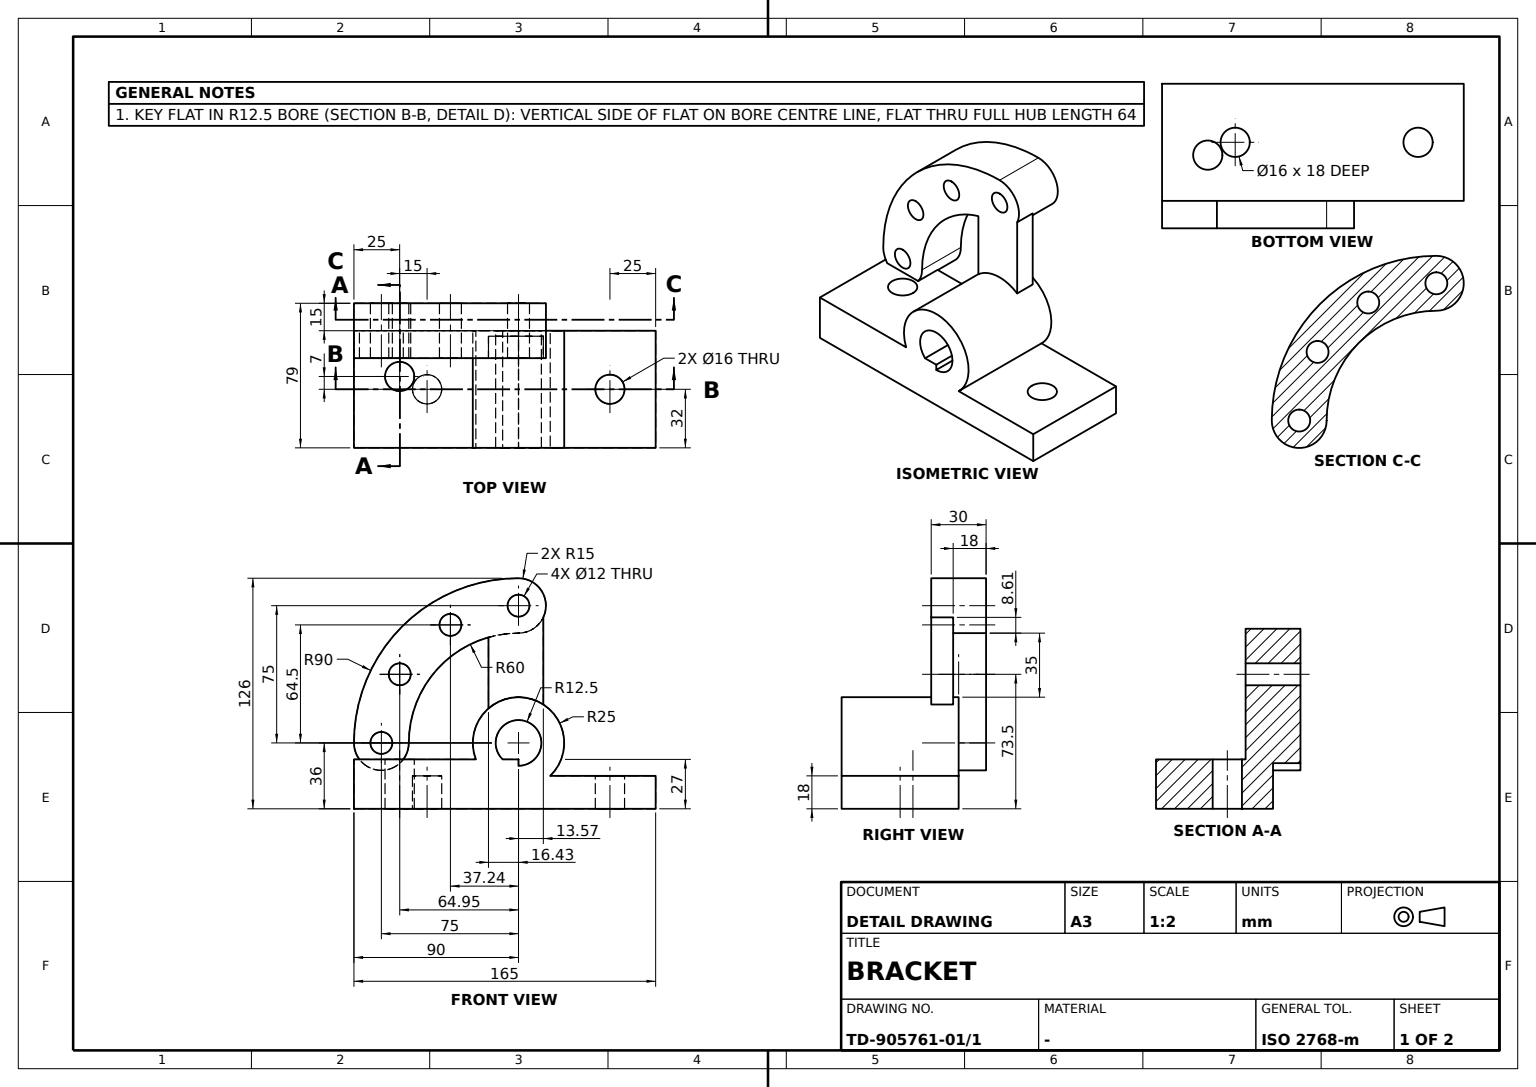
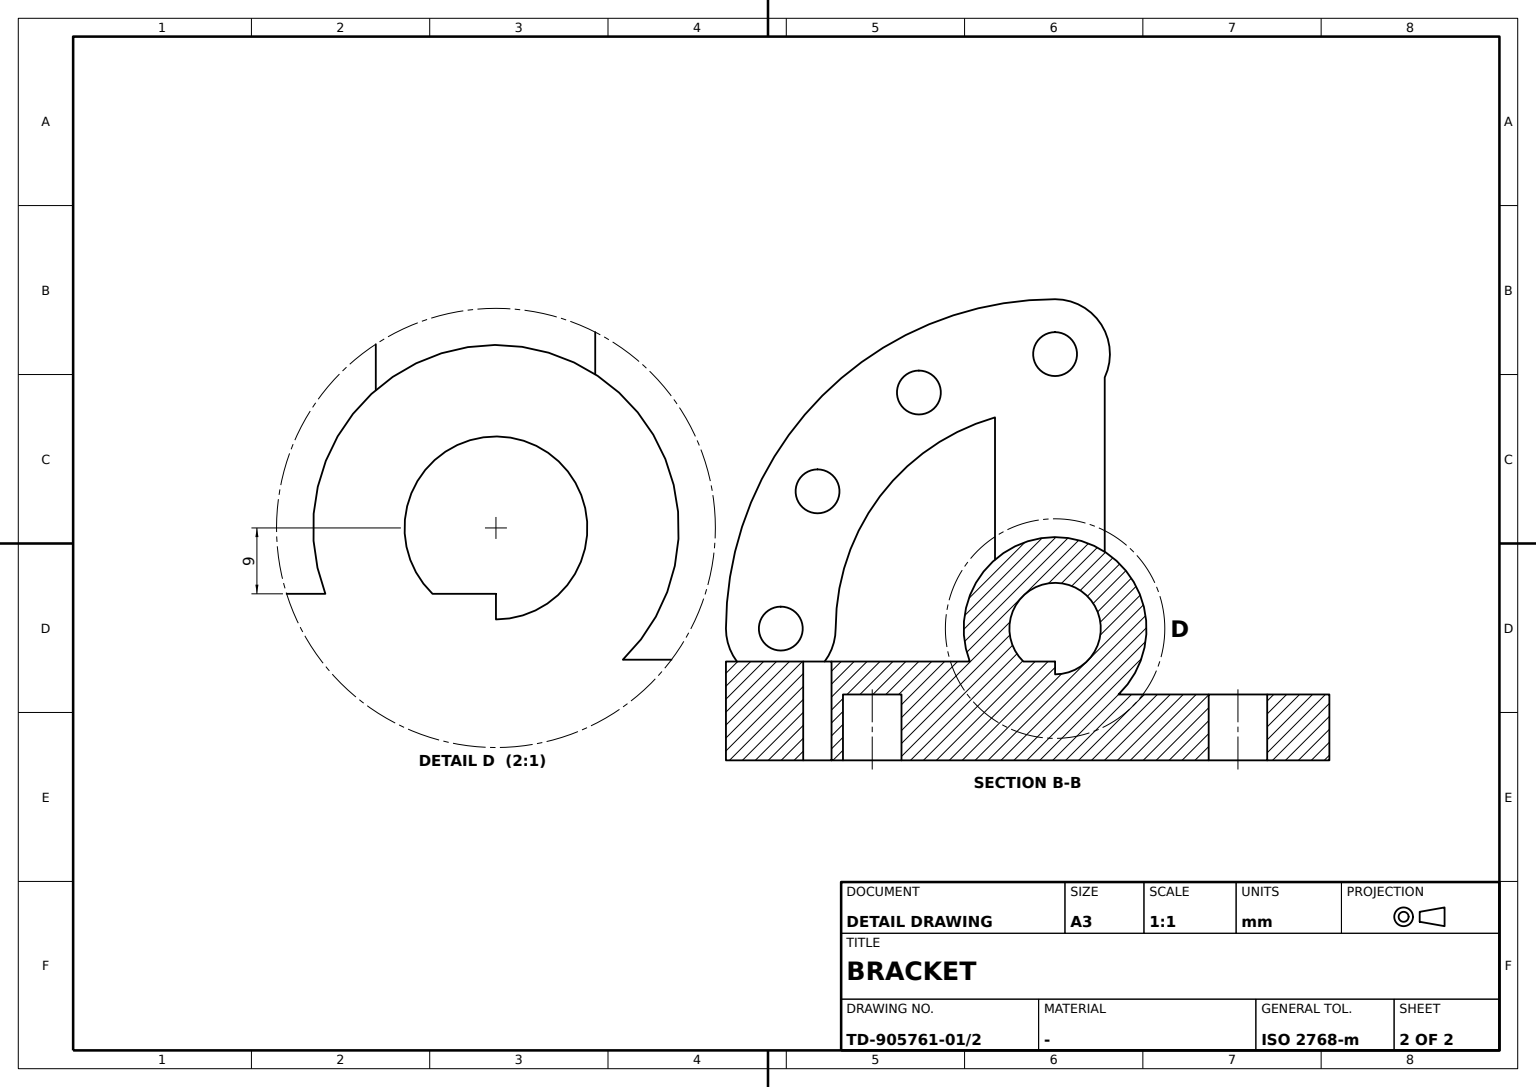
ISO-10303-21;
HEADER;
FILE_DESCRIPTION((''),'2;1');
FILE_NAME('','',(''),(''),'','','');
FILE_SCHEMA(('AUTOMOTIVE_DESIGN'));
ENDSEC;
DATA;
#1=APPLICATION_CONTEXT('');
#2=PRODUCT_CONTEXT('',#1,'mechanical');
#3=PRODUCT('','','',(#2));
#4=PRODUCT_DEFINITION_FORMATION('','',#3);
#5=PRODUCT_DEFINITION_CONTEXT('',#1,'design');
#6=PRODUCT_DEFINITION('','',#4,#5);
#7=PRODUCT_DEFINITION_SHAPE('','',#6);
#8=(LENGTH_UNIT()NAMED_UNIT(*)SI_UNIT(.MILLI.,.METRE.));
#9=(NAMED_UNIT(*)PLANE_ANGLE_UNIT()SI_UNIT($,.RADIAN.));
#10=(NAMED_UNIT(*)SI_UNIT($,.STERADIAN.)SOLID_ANGLE_UNIT());
#11=UNCERTAINTY_MEASURE_WITH_UNIT(LENGTH_MEASURE(0.005),#8,'distance_accuracy_value','');
#12=(GEOMETRIC_REPRESENTATION_CONTEXT(3)GLOBAL_UNCERTAINTY_ASSIGNED_CONTEXT((#11))GLOBAL_UNIT_ASSIGNED_CONTEXT((#8,#9,#10))REPRESENTATION_CONTEXT('',''));
#13=CARTESIAN_POINT('',(-16.427137,29.,57.707445));
#14=VERTEX_POINT('',#13);
#15=CARTESIAN_POINT('',(-16.427137,29.,18.845402));
#16=VERTEX_POINT('',#15);
#17=DIRECTION('',(0.,0.,-1.));
#18=VECTOR('',#17,1000.);
#19=LINE('',#13,#18);
#20=EDGE_CURVE('',#14,#16,#19,.T.);
#21=ORIENTED_EDGE('',*,*,#20,.F.);
#22=CARTESIAN_POINT('',(0.,29.,60.));
#23=VERTEX_POINT('',#22);
#24=CARTESIAN_POINT('',(0.,29.,0.));
#25=DIRECTION('',(0.,-1.,0.));
#26=AXIS2_PLACEMENT_3D('',#24,#25,#17);
#27=CIRCLE('',#26,60.);
#28=EDGE_CURVE('',#23,#14,#27,.T.);
#29=ORIENTED_EDGE('',*,*,#28,.F.);
#30=CARTESIAN_POINT('',(13.572863,29.,68.614283));
#31=VERTEX_POINT('',#30);
#32=CARTESIAN_POINT('',(0.,29.,75.));
#33=AXIS2_PLACEMENT_3D('',#32,#25,#17);
#34=CIRCLE('',#33,15.);
#35=EDGE_CURVE('',#23,#31,#34,.T.);
#36=ORIENTED_EDGE('',*,*,#35,.T.);
#37=CARTESIAN_POINT('',(13.572863,29.,20.994699));
#38=VERTEX_POINT('',#37);
#39=LINE('',#30,#18);
#40=EDGE_CURVE('',#31,#38,#39,.T.);
#41=ORIENTED_EDGE('',*,*,#40,.T.);
#42=CIRCLE('',#26,25.);
#43=EDGE_CURVE('',#38,#16,#42,.T.);
#44=ORIENTED_EDGE('',*,*,#43,.T.);
#45=EDGE_LOOP('',(#21,#29,#36,#41,#44));
#46=FACE_BOUND('',#45,.T.);
#47=DIRECTION('',(1.,0.,0.));
#48=AXIS2_PLACEMENT_3D('',#24,#25,#47);
#49=PLANE('',#48);
#50=ADVANCED_FACE('',(#46),#49,.F.);
#51=ORIENTED_EDGE('',*,*,#28,.T.);
#52=CARTESIAN_POINT('',(-16.427137,17.,57.707445));
#53=VERTEX_POINT('',#52);
#54=DIRECTION('',(0.,1.,0.));
#55=VECTOR('',#54,1000.);
#56=LINE('',#52,#55);
#57=EDGE_CURVE('',#53,#14,#56,.T.);
#58=ORIENTED_EDGE('',*,*,#57,.F.);
#59=CARTESIAN_POINT('',(-60.,17.,0.));
#60=VERTEX_POINT('',#59);
#61=CARTESIAN_POINT('',(0.,17.,0.));
#62=DIRECTION('',(0.,0.,1.));
#63=AXIS2_PLACEMENT_3D('',#61,#54,#62);
#64=CIRCLE('',#63,60.);
#65=EDGE_CURVE('',#60,#53,#64,.T.);
#66=ORIENTED_EDGE('',*,*,#65,.F.);
#67=CARTESIAN_POINT('',(-60.,47.,0.));
#68=VERTEX_POINT('',#67);
#69=CARTESIAN_POINT('',(-60.,32.,0.));
#70=LINE('',#69,#55);
#71=EDGE_CURVE('',#60,#68,#70,.T.);
#72=ORIENTED_EDGE('',*,*,#71,.T.);
#73=CARTESIAN_POINT('',(0.,47.,60.));
#74=VERTEX_POINT('',#73);
#75=CARTESIAN_POINT('',(0.,47.,0.));
#76=AXIS2_PLACEMENT_3D('',#75,#54,#62);
#77=CIRCLE('',#76,60.);
#78=EDGE_CURVE('',#68,#74,#77,.T.);
#79=ORIENTED_EDGE('',*,*,#78,.T.);
#80=CARTESIAN_POINT('',(0.,38.,60.));
#81=LINE('',#80,#55);
#82=EDGE_CURVE('',#23,#74,#81,.T.);
#83=ORIENTED_EDGE('',*,*,#82,.F.);
#84=EDGE_LOOP('',(#51,#58,#66,#72,#79,#83));
#85=FACE_BOUND('',#84,.T.);
#86=CARTESIAN_POINT('',(0.,32.,0.));
#87=DIRECTION('',(-1.,0.,0.));
#88=AXIS2_PLACEMENT_3D('',#86,#54,#87);
#89=CYLINDRICAL_SURFACE('',#88,60.);
#90=ADVANCED_FACE('',(#85),#89,.F.);
#91=CARTESIAN_POINT('',(-37.239092,17.,70.5));
#92=VERTEX_POINT('',#91);
#93=CARTESIAN_POINT('',(-37.239092,17.,64.5));
#94=AXIS2_PLACEMENT_3D('',#93,#54,#62);
#95=CIRCLE('',#94,6.);
#96=EDGE_CURVE('',#92,#92,#95,.T.);
#97=ORIENTED_EDGE('',*,*,#96,.F.);
#98=EDGE_LOOP('',(#97));
#99=FACE_BOUND('',#98,.T.);
#100=CARTESIAN_POINT('',(-37.239092,47.,70.5));
#101=VERTEX_POINT('',#100);
#102=CARTESIAN_POINT('',(-37.239092,47.,64.5));
#103=AXIS2_PLACEMENT_3D('',#102,#54,#62);
#104=CIRCLE('',#103,6.);
#105=EDGE_CURVE('',#101,#101,#104,.T.);
#106=ORIENTED_EDGE('',*,*,#105,.T.);
#107=EDGE_LOOP('',(#106));
#108=FACE_BOUND('',#107,.T.);
#109=CARTESIAN_POINT('',(-37.239092,32.,64.5));
#110=AXIS2_PLACEMENT_3D('',#109,#54,#87);
#111=CYLINDRICAL_SURFACE('',#110,6.);
#112=ADVANCED_FACE('',(#99,#108),#111,.F.);
#113=CARTESIAN_POINT('',(42.,0.,-18.));
#114=VERTEX_POINT('',#113);
#115=CARTESIAN_POINT('',(50.,0.,-18.));
#116=AXIS2_PLACEMENT_3D('',#115,#17,#87);
#117=CIRCLE('',#116,8.);
#118=EDGE_CURVE('',#114,#114,#117,.F.);
#119=ORIENTED_EDGE('',*,*,#118,.T.);
#120=EDGE_LOOP('',(#119));
#121=FACE_BOUND('',#120,.T.);
#122=CARTESIAN_POINT('',(58.,0.,-36.));
#123=VERTEX_POINT('',#122);
#124=CARTESIAN_POINT('',(50.,0.,-36.));
#125=AXIS2_PLACEMENT_3D('',#124,#62,#47);
#126=CIRCLE('',#125,8.);
#127=EDGE_CURVE('',#123,#123,#126,.T.);
#128=ORIENTED_EDGE('',*,*,#127,.F.);
#129=EDGE_LOOP('',(#128));
#130=FACE_BOUND('',#129,.T.);
#131=CARTESIAN_POINT('',(50.,0.,-27.66));
#132=AXIS2_PLACEMENT_3D('',#131,#62,#47);
#133=CYLINDRICAL_SURFACE('',#132,8.);
#134=ADVANCED_FACE('',(#121,#130),#133,.F.);
#135=CARTESIAN_POINT('',(0.,-32.,-12.5));
#136=VERTEX_POINT('',#135);
#137=CARTESIAN_POINT('',(0.,32.,-12.5));
#138=VERTEX_POINT('',#137);
#139=LINE('',#135,#55);
#140=EDGE_CURVE('',#136,#138,#139,.T.);
#141=ORIENTED_EDGE('',*,*,#140,.T.);
#142=CARTESIAN_POINT('',(0.,32.,-9.));
#143=VERTEX_POINT('',#142);
#144=LINE('',#86,#18);
#145=EDGE_CURVE('',#143,#138,#144,.T.);
#146=ORIENTED_EDGE('',*,*,#145,.F.);
#147=CARTESIAN_POINT('',(0.,-32.,-9.));
#148=VERTEX_POINT('',#147);
#149=CARTESIAN_POINT('',(0.,0.,-9.));
#150=LINE('',#149,#55);
#151=EDGE_CURVE('',#148,#143,#150,.T.);
#152=ORIENTED_EDGE('',*,*,#151,.F.);
#153=CARTESIAN_POINT('',(0.,-32.,0.));
#154=LINE('',#153,#18);
#155=EDGE_CURVE('',#148,#136,#154,.T.);
#156=ORIENTED_EDGE('',*,*,#155,.T.);
#157=EDGE_LOOP('',(#141,#146,#152,#156));
#158=FACE_BOUND('',#157,.T.);
#159=CARTESIAN_POINT('',(0.,0.,-18.));
#160=AXIS2_PLACEMENT_3D('',#159,#47,#17);
#161=PLANE('',#160);
#162=ADVANCED_FACE('',(#158),#161,.T.);
#163=CARTESIAN_POINT('',(-16.427137,17.,18.845402));
#164=VERTEX_POINT('',#163);
#165=CARTESIAN_POINT('',(-16.427137,17.,0.));
#166=LINE('',#165,#18);
#167=EDGE_CURVE('',#53,#164,#166,.T.);
#168=ORIENTED_EDGE('',*,*,#167,.F.);
#169=ORIENTED_EDGE('',*,*,#57,.T.);
#170=ORIENTED_EDGE('',*,*,#20,.T.);
#171=LINE('',#163,#55);
#172=EDGE_CURVE('',#164,#16,#171,.T.);
#173=ORIENTED_EDGE('',*,*,#172,.F.);
#174=EDGE_LOOP('',(#168,#169,#170,#173));
#175=FACE_BOUND('',#174,.T.);
#176=AXIS2_PLACEMENT_3D('',#52,#47,#17);
#177=PLANE('',#176);
#178=ADVANCED_FACE('',(#175),#177,.F.);
#179=CARTESIAN_POINT('',(-58.,0.,-18.));
#180=VERTEX_POINT('',#179);
#181=CARTESIAN_POINT('',(-50.,0.,-18.));
#182=AXIS2_PLACEMENT_3D('',#181,#17,#87);
#183=CIRCLE('',#182,8.);
#184=EDGE_CURVE('',#180,#180,#183,.T.);
#185=ORIENTED_EDGE('',*,*,#184,.T.);
#186=EDGE_LOOP('',(#185));
#187=FACE_BOUND('',#186,.T.);
#188=CARTESIAN_POINT('',(75.,0.,-18.));
#189=AXIS2_PLACEMENT_3D('',#188,#17,#87);
#190=PLANE('',#189);
#191=ADVANCED_FACE('',(#187),#190,.T.);
#192=CARTESIAN_POINT('',(-64.951905,47.,43.5));
#193=VERTEX_POINT('',#192);
#194=CARTESIAN_POINT('',(-64.951905,47.,37.5));
#195=AXIS2_PLACEMENT_3D('',#194,#54,#62);
#196=CIRCLE('',#195,6.);
#197=EDGE_CURVE('',#193,#193,#196,.T.);
#198=ORIENTED_EDGE('',*,*,#197,.T.);
#199=EDGE_LOOP('',(#198));
#200=FACE_BOUND('',#199,.T.);
#201=CARTESIAN_POINT('',(-64.951905,17.,43.5));
#202=VERTEX_POINT('',#201);
#203=CARTESIAN_POINT('',(-64.951905,17.,37.5));
#204=AXIS2_PLACEMENT_3D('',#203,#54,#62);
#205=CIRCLE('',#204,6.);
#206=EDGE_CURVE('',#202,#202,#205,.T.);
#207=ORIENTED_EDGE('',*,*,#206,.F.);
#208=EDGE_LOOP('',(#207));
#209=FACE_BOUND('',#208,.T.);
#210=CARTESIAN_POINT('',(-64.951905,32.,37.5));
#211=AXIS2_PLACEMENT_3D('',#210,#54,#87);
#212=CYLINDRICAL_SURFACE('',#211,6.);
#213=ADVANCED_FACE('',(#200,#209),#212,.F.);
#214=CARTESIAN_POINT('',(-63.,17.,-9.));
#215=VERTEX_POINT('',#214);
#216=CARTESIAN_POINT('',(-63.,32.,-9.));
#217=VERTEX_POINT('',#216);
#218=LINE('',#216,#55);
#219=EDGE_CURVE('',#215,#217,#218,.T.);
#220=ORIENTED_EDGE('',*,*,#219,.F.);
#221=CARTESIAN_POINT('',(-87.,17.,-9.));
#222=VERTEX_POINT('',#221);
#223=CARTESIAN_POINT('',(0.,17.,-9.));
#224=VECTOR('',#47,1000.);
#225=LINE('',#223,#224);
#226=EDGE_CURVE('',#222,#215,#225,.T.);
#227=ORIENTED_EDGE('',*,*,#226,.F.);
#228=CARTESIAN_POINT('',(-87.,32.,-9.));
#229=VERTEX_POINT('',#228);
#230=LINE('',#228,#55);
#231=EDGE_CURVE('',#229,#222,#230,.F.);
#232=ORIENTED_EDGE('',*,*,#231,.F.);
#233=CARTESIAN_POINT('',(-90.,32.,-9.));
#234=VERTEX_POINT('',#233);
#235=LINE('',#142,#224);
#236=EDGE_CURVE('',#234,#229,#235,.T.);
#237=ORIENTED_EDGE('',*,*,#236,.F.);
#238=CARTESIAN_POINT('',(-90.,-32.,-9.));
#239=VERTEX_POINT('',#238);
#240=CARTESIAN_POINT('',(-90.,0.,-9.));
#241=LINE('',#240,#55);
#242=EDGE_CURVE('',#239,#234,#241,.T.);
#243=ORIENTED_EDGE('',*,*,#242,.F.);
#244=CARTESIAN_POINT('',(-23.323808,-32.,-9.));
#245=VERTEX_POINT('',#244);
#246=LINE('',#147,#224);
#247=EDGE_CURVE('',#239,#245,#246,.T.);
#248=ORIENTED_EDGE('',*,*,#247,.T.);
#249=CARTESIAN_POINT('',(-23.323808,32.,-9.));
#250=VERTEX_POINT('',#249);
#251=LINE('',#244,#55);
#252=EDGE_CURVE('',#245,#250,#251,.T.);
#253=ORIENTED_EDGE('',*,*,#252,.T.);
#254=EDGE_CURVE('',#217,#250,#235,.T.);
#255=ORIENTED_EDGE('',*,*,#254,.F.);
#256=EDGE_LOOP('',(#220,#227,#232,#237,#243,#248,#253,#255));
#257=FACE_BOUND('',#256,.T.);
#258=CARTESIAN_POINT('',(-57.,7.,-9.));
#259=VERTEX_POINT('',#258);
#260=CARTESIAN_POINT('',(-65.,7.,-9.));
#261=AXIS2_PLACEMENT_3D('',#260,#62,#47);
#262=CIRCLE('',#261,8.);
#263=EDGE_CURVE('',#259,#259,#262,.T.);
#264=ORIENTED_EDGE('',*,*,#263,.F.);
#265=EDGE_LOOP('',(#264));
#266=FACE_BOUND('',#265,.T.);
#267=AXIS2_PLACEMENT_3D('',#240,#62,#47);
#268=PLANE('',#267);
#269=ADVANCED_FACE('',(#257,#266),#268,.T.);
#270=CARTESIAN_POINT('',(-75.,17.,6.));
#271=VERTEX_POINT('',#270);
#272=CARTESIAN_POINT('',(-75.,17.,0.));
#273=AXIS2_PLACEMENT_3D('',#272,#54,#62);
#274=CIRCLE('',#273,6.);
#275=EDGE_CURVE('',#271,#271,#274,.T.);
#276=ORIENTED_EDGE('',*,*,#275,.F.);
#277=EDGE_LOOP('',(#276));
#278=FACE_BOUND('',#277,.T.);
#279=CARTESIAN_POINT('',(-75.,47.,6.));
#280=VERTEX_POINT('',#279);
#281=CARTESIAN_POINT('',(-75.,47.,0.));
#282=AXIS2_PLACEMENT_3D('',#281,#54,#62);
#283=CIRCLE('',#282,6.);
#284=EDGE_CURVE('',#280,#280,#283,.T.);
#285=ORIENTED_EDGE('',*,*,#284,.T.);
#286=EDGE_LOOP('',(#285));
#287=FACE_BOUND('',#286,.T.);
#288=CARTESIAN_POINT('',(-75.,32.,0.));
#289=AXIS2_PLACEMENT_3D('',#288,#54,#87);
#290=CYLINDRICAL_SURFACE('',#289,6.);
#291=ADVANCED_FACE('',(#278,#287),#290,.F.);
#292=CARTESIAN_POINT('',(13.572863,17.,20.994699));
#293=VERTEX_POINT('',#292);
#294=LINE('',#292,#55);
#295=EDGE_CURVE('',#293,#38,#294,.T.);
#296=ORIENTED_EDGE('',*,*,#295,.F.);
#297=CIRCLE('',#63,25.);
#298=EDGE_CURVE('',#293,#164,#297,.F.);
#299=ORIENTED_EDGE('',*,*,#298,.T.);
#300=ORIENTED_EDGE('',*,*,#172,.T.);
#301=ORIENTED_EDGE('',*,*,#43,.F.);
#302=EDGE_LOOP('',(#296,#299,#300,#301));
#303=FACE_BOUND('',#302,.T.);
#304=ORIENTED_EDGE('',*,*,#252,.F.);
#305=CARTESIAN_POINT('',(17.349352,-32.,-18.));
#306=VERTEX_POINT('',#305);
#307=AXIS2_PLACEMENT_3D('',#153,#54,#62);
#308=CIRCLE('',#307,25.);
#309=EDGE_CURVE('',#245,#306,#308,.T.);
#310=ORIENTED_EDGE('',*,*,#309,.T.);
#311=CARTESIAN_POINT('',(17.349352,32.,-18.));
#312=VERTEX_POINT('',#311);
#313=LINE('',#305,#55);
#314=EDGE_CURVE('',#306,#312,#313,.T.);
#315=ORIENTED_EDGE('',*,*,#314,.T.);
#316=AXIS2_PLACEMENT_3D('',#86,#54,#62);
#317=CIRCLE('',#316,25.);
#318=EDGE_CURVE('',#250,#312,#317,.T.);
#319=ORIENTED_EDGE('',*,*,#318,.F.);
#320=EDGE_LOOP('',(#304,#310,#315,#319));
#321=FACE_BOUND('',#320,.T.);
#322=CARTESIAN_POINT('',(0.,0.,0.));
#323=AXIS2_PLACEMENT_3D('',#322,#54,#87);
#324=CYLINDRICAL_SURFACE('',#323,25.);
#325=ADVANCED_FACE('',(#303,#321),#324,.T.);
#326=CARTESIAN_POINT('',(0.,17.,81.));
#327=VERTEX_POINT('',#326);
#328=CARTESIAN_POINT('',(0.,17.,75.));
#329=AXIS2_PLACEMENT_3D('',#328,#54,#62);
#330=CIRCLE('',#329,6.);
#331=EDGE_CURVE('',#327,#327,#330,.T.);
#332=ORIENTED_EDGE('',*,*,#331,.T.);
#333=EDGE_LOOP('',(#332));
#334=FACE_BOUND('',#333,.T.);
#335=ORIENTED_EDGE('',*,*,#65,.T.);
#336=ORIENTED_EDGE('',*,*,#167,.T.);
#337=ORIENTED_EDGE('',*,*,#298,.F.);
#338=CARTESIAN_POINT('',(13.572863,17.,68.614283));
#339=VERTEX_POINT('',#338);
#340=CARTESIAN_POINT('',(13.572863,17.,0.));
#341=LINE('',#340,#18);
#342=EDGE_CURVE('',#339,#293,#341,.T.);
#343=ORIENTED_EDGE('',*,*,#342,.F.);
#344=CARTESIAN_POINT('',(0.,17.,90.));
#345=VERTEX_POINT('',#344);
#346=CIRCLE('',#329,15.);
#347=EDGE_CURVE('',#345,#339,#346,.T.);
#348=ORIENTED_EDGE('',*,*,#347,.F.);
#349=CARTESIAN_POINT('',(-90.,17.,0.));
#350=VERTEX_POINT('',#349);
#351=CIRCLE('',#63,90.);
#352=EDGE_CURVE('',#350,#345,#351,.T.);
#353=ORIENTED_EDGE('',*,*,#352,.F.);
#354=CIRCLE('',#273,15.);
#355=EDGE_CURVE('',#222,#350,#354,.T.);
#356=ORIENTED_EDGE('',*,*,#355,.F.);
#357=ORIENTED_EDGE('',*,*,#226,.T.);
#358=EDGE_CURVE('',#60,#215,#354,.T.);
#359=ORIENTED_EDGE('',*,*,#358,.F.);
#360=EDGE_LOOP('',(#335,#336,#337,#343,#348,#353,#356,#357,#359));
#361=FACE_BOUND('',#360,.T.);
#362=ORIENTED_EDGE('',*,*,#206,.T.);
#363=EDGE_LOOP('',(#362));
#364=FACE_BOUND('',#363,.T.);
#365=ORIENTED_EDGE('',*,*,#96,.T.);
#366=EDGE_LOOP('',(#365));
#367=FACE_BOUND('',#366,.T.);
#368=ORIENTED_EDGE('',*,*,#275,.T.);
#369=EDGE_LOOP('',(#368));
#370=FACE_BOUND('',#369,.T.);
#371=AXIS2_PLACEMENT_3D('',#61,#54,#87);
#372=PLANE('',#371);
#373=ADVANCED_FACE('',(#334,#361,#364,#367,#370),#372,.F.);
#374=CARTESIAN_POINT('',(-42.,0.,-36.));
#375=VERTEX_POINT('',#374);
#376=CARTESIAN_POINT('',(-50.,0.,-36.));
#377=AXIS2_PLACEMENT_3D('',#376,#62,#47);
#378=CIRCLE('',#377,8.);
#379=EDGE_CURVE('',#375,#375,#378,.T.);
#380=ORIENTED_EDGE('',*,*,#379,.T.);
#381=EDGE_LOOP('',(#380));
#382=FACE_BOUND('',#381,.T.);
#383=CARTESIAN_POINT('',(-57.,7.,-36.));
#384=VERTEX_POINT('',#383);
#385=CARTESIAN_POINT('',(-65.,7.,-36.));
#386=AXIS2_PLACEMENT_3D('',#385,#62,#47);
#387=CIRCLE('',#386,8.);
#388=EDGE_CURVE('',#384,#384,#387,.T.);
#389=ORIENTED_EDGE('',*,*,#388,.T.);
#390=EDGE_LOOP('',(#389));
#391=FACE_BOUND('',#390,.T.);
#392=CARTESIAN_POINT('',(-90.,32.,-36.));
#393=VERTEX_POINT('',#392);
#394=CARTESIAN_POINT('',(75.,32.,-36.));
#395=VERTEX_POINT('',#394);
#396=CARTESIAN_POINT('',(0.,32.,-36.));
#397=LINE('',#396,#224);
#398=EDGE_CURVE('',#393,#395,#397,.T.);
#399=ORIENTED_EDGE('',*,*,#398,.T.);
#400=CARTESIAN_POINT('',(75.,-32.,-36.));
#401=VERTEX_POINT('',#400);
#402=CARTESIAN_POINT('',(75.,0.,-36.));
#403=LINE('',#402,#55);
#404=EDGE_CURVE('',#401,#395,#403,.T.);
#405=ORIENTED_EDGE('',*,*,#404,.F.);
#406=CARTESIAN_POINT('',(-90.,-32.,-36.));
#407=VERTEX_POINT('',#406);
#408=CARTESIAN_POINT('',(0.,-32.,-36.));
#409=LINE('',#408,#224);
#410=EDGE_CURVE('',#407,#401,#409,.T.);
#411=ORIENTED_EDGE('',*,*,#410,.F.);
#412=CARTESIAN_POINT('',(-90.,0.,-36.));
#413=LINE('',#412,#55);
#414=EDGE_CURVE('',#407,#393,#413,.T.);
#415=ORIENTED_EDGE('',*,*,#414,.T.);
#416=EDGE_LOOP('',(#399,#405,#411,#415));
#417=FACE_BOUND('',#416,.T.);
#418=ORIENTED_EDGE('',*,*,#127,.T.);
#419=EDGE_LOOP('',(#418));
#420=FACE_BOUND('',#419,.T.);
#421=CARTESIAN_POINT('',(0.,0.,-36.));
#422=AXIS2_PLACEMENT_3D('',#421,#62,#47);
#423=PLANE('',#422);
#424=ADVANCED_FACE('',(#382,#391,#417,#420),#423,.F.);
#425=ORIENTED_EDGE('',*,*,#236,.T.);
#426=AXIS2_PLACEMENT_3D('',#288,#54,#62);
#427=CIRCLE('',#426,15.);
#428=EDGE_CURVE('',#217,#229,#427,.T.);
#429=ORIENTED_EDGE('',*,*,#428,.F.);
#430=ORIENTED_EDGE('',*,*,#254,.T.);
#431=ORIENTED_EDGE('',*,*,#318,.T.);
#432=CARTESIAN_POINT('',(75.,32.,-18.));
#433=VERTEX_POINT('',#432);
#434=CARTESIAN_POINT('',(0.,32.,-18.));
#435=VECTOR('',#87,1000.);
#436=LINE('',#434,#435);
#437=EDGE_CURVE('',#433,#312,#436,.T.);
#438=ORIENTED_EDGE('',*,*,#437,.F.);
#439=CARTESIAN_POINT('',(75.,32.,0.));
#440=VECTOR('',#62,1000.);
#441=LINE('',#439,#440);
#442=EDGE_CURVE('',#395,#433,#441,.T.);
#443=ORIENTED_EDGE('',*,*,#442,.F.);
#444=ORIENTED_EDGE('',*,*,#398,.F.);
#445=CARTESIAN_POINT('',(-90.,32.,0.));
#446=LINE('',#445,#440);
#447=EDGE_CURVE('',#393,#234,#446,.T.);
#448=ORIENTED_EDGE('',*,*,#447,.T.);
#449=EDGE_LOOP('',(#425,#429,#430,#431,#438,#443,#444,#448));
#450=FACE_BOUND('',#449,.T.);
#451=ORIENTED_EDGE('',*,*,#145,.T.);
#452=CARTESIAN_POINT('',(-8.674676,32.,-9.));
#453=VERTEX_POINT('',#452);
#454=CIRCLE('',#316,12.5);
#455=EDGE_CURVE('',#453,#138,#454,.T.);
#456=ORIENTED_EDGE('',*,*,#455,.F.);
#457=EDGE_CURVE('',#453,#143,#235,.T.);
#458=ORIENTED_EDGE('',*,*,#457,.T.);
#459=EDGE_LOOP('',(#451,#456,#458));
#460=FACE_BOUND('',#459,.T.);
#461=PLANE('',#88);
#462=ADVANCED_FACE('',(#450,#460),#461,.T.);
#463=ORIENTED_EDGE('',*,*,#442,.T.);
#464=CARTESIAN_POINT('',(75.,-32.,-18.));
#465=VERTEX_POINT('',#464);
#466=LINE('',#188,#55);
#467=EDGE_CURVE('',#465,#433,#466,.T.);
#468=ORIENTED_EDGE('',*,*,#467,.F.);
#469=CARTESIAN_POINT('',(75.,-32.,0.));
#470=LINE('',#469,#440);
#471=EDGE_CURVE('',#401,#465,#470,.T.);
#472=ORIENTED_EDGE('',*,*,#471,.F.);
#473=ORIENTED_EDGE('',*,*,#404,.T.);
#474=EDGE_LOOP('',(#463,#468,#472,#473));
#475=FACE_BOUND('',#474,.T.);
#476=AXIS2_PLACEMENT_3D('',#402,#87,#62);
#477=PLANE('',#476);
#478=ADVANCED_FACE('',(#475),#477,.F.);
#479=ORIENTED_EDGE('',*,*,#140,.F.);
#480=CARTESIAN_POINT('',(-8.674676,-32.,-9.));
#481=VERTEX_POINT('',#480);
#482=CIRCLE('',#307,12.5);
#483=EDGE_CURVE('',#481,#136,#482,.T.);
#484=ORIENTED_EDGE('',*,*,#483,.F.);
#485=LINE('',#480,#55);
#486=EDGE_CURVE('',#481,#453,#485,.T.);
#487=ORIENTED_EDGE('',*,*,#486,.T.);
#488=ORIENTED_EDGE('',*,*,#455,.T.);
#489=EDGE_LOOP('',(#479,#484,#487,#488));
#490=FACE_BOUND('',#489,.T.);
#491=CYLINDRICAL_SURFACE('',#323,12.5);
#492=ADVANCED_FACE('',(#490),#491,.F.);
#493=LINE('',#338,#55);
#494=EDGE_CURVE('',#339,#31,#493,.T.);
#495=ORIENTED_EDGE('',*,*,#494,.F.);
#496=ORIENTED_EDGE('',*,*,#342,.T.);
#497=ORIENTED_EDGE('',*,*,#295,.T.);
#498=ORIENTED_EDGE('',*,*,#40,.F.);
#499=EDGE_LOOP('',(#495,#496,#497,#498));
#500=FACE_BOUND('',#499,.T.);
#501=AXIS2_PLACEMENT_3D('',#338,#47,#17);
#502=PLANE('',#501);
#503=ADVANCED_FACE('',(#500),#502,.T.);
#504=ORIENTED_EDGE('',*,*,#263,.T.);
#505=EDGE_LOOP('',(#504));
#506=FACE_BOUND('',#505,.T.);
#507=ORIENTED_EDGE('',*,*,#388,.F.);
#508=EDGE_LOOP('',(#507));
#509=FACE_BOUND('',#508,.T.);
#510=CARTESIAN_POINT('',(-65.,7.,-23.16));
#511=AXIS2_PLACEMENT_3D('',#510,#62,#47);
#512=CYLINDRICAL_SURFACE('',#511,8.);
#513=ADVANCED_FACE('',(#506,#509),#512,.F.);
#514=CARTESIAN_POINT('',(-90.,47.,0.));
#515=VERTEX_POINT('',#514);
#516=CIRCLE('',#282,15.);
#517=EDGE_CURVE('',#68,#515,#516,.T.);
#518=ORIENTED_EDGE('',*,*,#517,.T.);
#519=CARTESIAN_POINT('',(0.,47.,90.));
#520=VERTEX_POINT('',#519);
#521=CIRCLE('',#76,90.);
#522=EDGE_CURVE('',#515,#520,#521,.T.);
#523=ORIENTED_EDGE('',*,*,#522,.T.);
#524=CARTESIAN_POINT('',(0.,47.,75.));
#525=AXIS2_PLACEMENT_3D('',#524,#54,#62);
#526=CIRCLE('',#525,15.);
#527=EDGE_CURVE('',#520,#74,#526,.T.);
#528=ORIENTED_EDGE('',*,*,#527,.T.);
#529=ORIENTED_EDGE('',*,*,#78,.F.);
#530=EDGE_LOOP('',(#518,#523,#528,#529));
#531=FACE_BOUND('',#530,.T.);
#532=CARTESIAN_POINT('',(0.,47.,81.));
#533=VERTEX_POINT('',#532);
#534=CIRCLE('',#525,6.);
#535=EDGE_CURVE('',#533,#533,#534,.T.);
#536=ORIENTED_EDGE('',*,*,#535,.F.);
#537=EDGE_LOOP('',(#536));
#538=FACE_BOUND('',#537,.T.);
#539=ORIENTED_EDGE('',*,*,#284,.F.);
#540=EDGE_LOOP('',(#539));
#541=FACE_BOUND('',#540,.T.);
#542=ORIENTED_EDGE('',*,*,#197,.F.);
#543=EDGE_LOOP('',(#542));
#544=FACE_BOUND('',#543,.T.);
#545=ORIENTED_EDGE('',*,*,#105,.F.);
#546=EDGE_LOOP('',(#545));
#547=FACE_BOUND('',#546,.T.);
#548=AXIS2_PLACEMENT_3D('',#75,#54,#87);
#549=PLANE('',#548);
#550=ADVANCED_FACE('',(#531,#538,#541,#544,#547),#549,.T.);
#551=ORIENTED_EDGE('',*,*,#535,.T.);
#552=EDGE_LOOP('',(#551));
#553=FACE_BOUND('',#552,.T.);
#554=ORIENTED_EDGE('',*,*,#331,.F.);
#555=EDGE_LOOP('',(#554));
#556=FACE_BOUND('',#555,.T.);
#557=CARTESIAN_POINT('',(0.,32.,75.));
#558=AXIS2_PLACEMENT_3D('',#557,#54,#87);
#559=CYLINDRICAL_SURFACE('',#558,6.);
#560=ADVANCED_FACE('',(#553,#556),#559,.F.);
#561=LINE('',#445,#55);
#562=EDGE_CURVE('',#350,#515,#561,.T.);
#563=ORIENTED_EDGE('',*,*,#562,.F.);
#564=ORIENTED_EDGE('',*,*,#352,.T.);
#565=CARTESIAN_POINT('',(0.,32.,90.));
#566=LINE('',#565,#55);
#567=EDGE_CURVE('',#345,#520,#566,.T.);
#568=ORIENTED_EDGE('',*,*,#567,.T.);
#569=ORIENTED_EDGE('',*,*,#522,.F.);
#570=EDGE_LOOP('',(#563,#564,#568,#569));
#571=FACE_BOUND('',#570,.T.);
#572=CYLINDRICAL_SURFACE('',#88,90.);
#573=ADVANCED_FACE('',(#571),#572,.T.);
#574=ORIENTED_EDGE('',*,*,#118,.F.);
#575=EDGE_LOOP('',(#574));
#576=FACE_BOUND('',#575,.T.);
#577=ORIENTED_EDGE('',*,*,#437,.T.);
#578=ORIENTED_EDGE('',*,*,#314,.F.);
#579=CARTESIAN_POINT('',(0.,-32.,-18.));
#580=LINE('',#579,#435);
#581=EDGE_CURVE('',#465,#306,#580,.T.);
#582=ORIENTED_EDGE('',*,*,#581,.F.);
#583=ORIENTED_EDGE('',*,*,#467,.T.);
#584=EDGE_LOOP('',(#577,#578,#582,#583));
#585=FACE_BOUND('',#584,.T.);
#586=ADVANCED_FACE('',(#576,#585),#190,.F.);
#587=ORIENTED_EDGE('',*,*,#483,.T.);
#588=ORIENTED_EDGE('',*,*,#155,.F.);
#589=EDGE_CURVE('',#481,#148,#246,.T.);
#590=ORIENTED_EDGE('',*,*,#589,.F.);
#591=EDGE_LOOP('',(#587,#588,#590));
#592=FACE_BOUND('',#591,.T.);
#593=ORIENTED_EDGE('',*,*,#581,.T.);
#594=ORIENTED_EDGE('',*,*,#309,.F.);
#595=ORIENTED_EDGE('',*,*,#247,.F.);
#596=CARTESIAN_POINT('',(-90.,-32.,0.));
#597=LINE('',#596,#440);
#598=EDGE_CURVE('',#407,#239,#597,.T.);
#599=ORIENTED_EDGE('',*,*,#598,.F.);
#600=ORIENTED_EDGE('',*,*,#410,.T.);
#601=ORIENTED_EDGE('',*,*,#471,.T.);
#602=EDGE_LOOP('',(#593,#594,#595,#599,#600,#601));
#603=FACE_BOUND('',#602,.T.);
#604=AXIS2_PLACEMENT_3D('',#153,#54,#87);
#605=PLANE('',#604);
#606=ADVANCED_FACE('',(#592,#603),#605,.F.);
#607=ORIENTED_EDGE('',*,*,#457,.F.);
#608=ORIENTED_EDGE('',*,*,#486,.F.);
#609=ORIENTED_EDGE('',*,*,#589,.T.);
#610=ORIENTED_EDGE('',*,*,#151,.T.);
#611=EDGE_LOOP('',(#607,#608,#609,#610));
#612=FACE_BOUND('',#611,.T.);
#613=ADVANCED_FACE('',(#612),#268,.T.);
#614=ORIENTED_EDGE('',*,*,#184,.F.);
#615=EDGE_LOOP('',(#614));
#616=FACE_BOUND('',#615,.T.);
#617=ORIENTED_EDGE('',*,*,#379,.F.);
#618=EDGE_LOOP('',(#617));
#619=FACE_BOUND('',#618,.T.);
#620=CARTESIAN_POINT('',(-50.,0.,-27.66));
#621=AXIS2_PLACEMENT_3D('',#620,#17,#87);
#622=CYLINDRICAL_SURFACE('',#621,8.);
#623=ADVANCED_FACE('',(#616,#619),#622,.F.);
#624=ORIENTED_EDGE('',*,*,#219,.T.);
#625=ORIENTED_EDGE('',*,*,#428,.T.);
#626=ORIENTED_EDGE('',*,*,#231,.T.);
#627=ORIENTED_EDGE('',*,*,#355,.T.);
#628=ORIENTED_EDGE('',*,*,#562,.T.);
#629=ORIENTED_EDGE('',*,*,#517,.F.);
#630=ORIENTED_EDGE('',*,*,#71,.F.);
#631=ORIENTED_EDGE('',*,*,#358,.T.);
#632=EDGE_LOOP('',(#624,#625,#626,#627,#628,#629,#630,#631));
#633=FACE_BOUND('',#632,.T.);
#634=CYLINDRICAL_SURFACE('',#289,15.);
#635=ADVANCED_FACE('',(#633),#634,.T.);
#636=ORIENTED_EDGE('',*,*,#567,.F.);
#637=ORIENTED_EDGE('',*,*,#347,.T.);
#638=ORIENTED_EDGE('',*,*,#494,.T.);
#639=ORIENTED_EDGE('',*,*,#35,.F.);
#640=ORIENTED_EDGE('',*,*,#82,.T.);
#641=ORIENTED_EDGE('',*,*,#527,.F.);
#642=EDGE_LOOP('',(#636,#637,#638,#639,#640,#641));
#643=FACE_BOUND('',#642,.T.);
#644=CYLINDRICAL_SURFACE('',#558,15.);
#645=ADVANCED_FACE('',(#643),#644,.T.);
#646=ORIENTED_EDGE('',*,*,#598,.T.);
#647=ORIENTED_EDGE('',*,*,#242,.T.);
#648=ORIENTED_EDGE('',*,*,#447,.F.);
#649=ORIENTED_EDGE('',*,*,#414,.F.);
#650=EDGE_LOOP('',(#646,#647,#648,#649));
#651=FACE_BOUND('',#650,.T.);
#652=AXIS2_PLACEMENT_3D('',#412,#87,#62);
#653=PLANE('',#652);
#654=ADVANCED_FACE('',(#651),#653,.T.);
#655=CLOSED_SHELL('',(#50,#90,#112,#134,#162,#178,#191,#213,#269,#291,#325,#373,#424,#462,#478,#492,#503,#513,#550,#560,#573,#586,#606,#613,#623,#635,#645,#654));
#656=MANIFOLD_SOLID_BREP('',#655);
#657=ADVANCED_BREP_SHAPE_REPRESENTATION('',(#656),#12);
#658=SHAPE_DEFINITION_REPRESENTATION(#7,#657);
ENDSEC;
END-ISO-10303-21;
